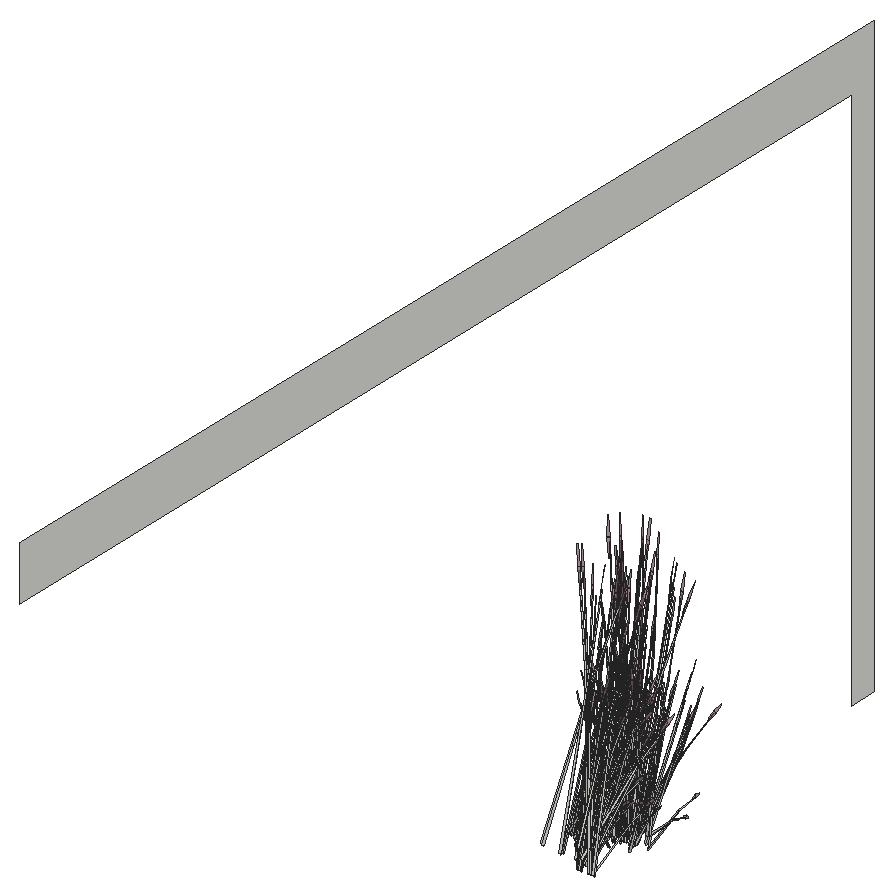
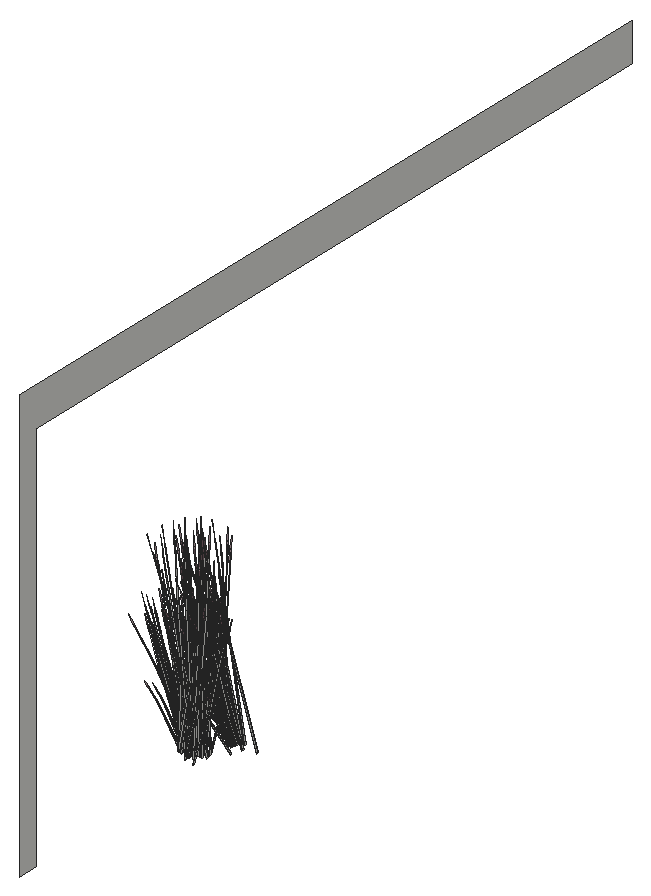
# SketchUp Ruby script. Lengths in inches.
U = 1.inch
M = Sketchup.active_model
def pt(a) = Geom::Point3d.new(a.map { |v| v * U })
def face(e, loops, mat)
  f = e.add_face(loops[0].map { |a| pt(a) })
  loops[1..].each { |l| e.add_face(l.map { |a| pt(a) }).erase! }
  f.material = f.back_material = mat if mat
  f
end
# faces: each face lists its corners as indices into pts; further lists are holes
def faces(e, pts, list, mat = nil) = list.each { |f| face(e, (f[0].is_a?(Array) ? f : [f]).map { |l| l.map { |i| pts[i] } }, mat) }
# xy, xz, yz: faces in a plane at the given z, y or x. An outline is a flat list of corners, or four numbers for a rectangle; further outlines are holes
def ring(l) = l.size == 4 ? [[l[0], l[1]], [l[2], l[1]], [l[2], l[3]], [l[0], l[3]]] : l.each_slice(2).to_a
def flat(e, list, mat, &to3) = list.each { |f| face(e, (f[0].is_a?(Array) ? f : [f]).map { |l| ring(l).map { |u, v| to3.(u, v) } }, mat) }
def xy(e, z, list, mat = nil) = flat(e, list, mat) { |x, y| [x, y, z] }
def xz(e, y, list, mat = nil) = flat(e, list, mat) { |x, z| [x, y, z] }
def yz(e, x, list, mat = nil) = flat(e, list, mat) { |y, z| [x, y, z] }
def lines(e, pts, list) = list.each { |a, b| e.add_line(pt(pts[a]), pt(pts[b])) }
# prism: a flat outline (further loops are holes) pulled along v
def prism(e, loops, v, mat = nil)
  f = face(e, loops, mat); d = Geom::Vector3d.new(v.map { |x| x * U })
  f.pushpull(f.normal.samedirection?(d) ? d.length : -d.length)
end
def box(e, o, s, mat = nil) = prism(e, [[o, [o[0] + s[0], o[1], o[2]], [o[0] + s[0], o[1] + s[1], o[2]], [o[0], o[1] + s[1], o[2]]]], [0, 0, s[2]], mat)
def at(x, y, z, deg = 0) = Geom::Transformation.translation(pt([x, y, z])) * Geom::Transformation.rotation(ORIGIN, Z_AXIS, deg.degrees)
def axes(o, x, y, z) = Geom::Transformation.new([*x, 0, *y, 0, *z, 0, *pt(o).to_a, 1])
def part(name) = M.definitions.add(name)
# library, detail: a bought-in or finely detailed component or shape, given as its bounding box
def library(name, o, s) = part(name).tap { |d| box(d.entities, o, s) }
def detail(e, o, s) = box(e.add_group.entities, o, s)
def put(e, d, t, mat = nil) = e.add_instance(d, t).tap { |i| i.material = mat if mat }
def group(e, t, mat = nil) = e.add_group.tap { |g| g.transformation = t; g.material = mat if mat }.entities
root = M.entities
M.materials.add("LightPink_Translucent").color = [144, 107, 117]
M.materials["LightPink_Translucent"].alpha = 0.75
c1 = part("blade")
p = [[2.15,0.21,22],[0,0.17,0],[0.09,0.45,0],[2.18,0.31,22],[2.29,0.31,22],[0.38,0.45,0],
  [2.48,0.24,33],[2.49,0.24,33],[2.48,0.22,33]]
faces(c1.entities,p,[[0,1,2,3],[4,5,2,3],[6,3,4,7],[8,0,3,6]])
c2 = part("seeds")
p = [[0.3,-0.1,1.38],[-0.01,-0.03,1.59],[-0.01,-0.03,0.03],[0.14,-0.07,-0.07],[0.29,-0.03,3],[0.15,0.01,3.11]]
faces(c2.entities,p,[[0,1,2,3],[1,0,4,5]],"LightPink_Translucent")
c3 = part("blade with seeds")
put(c3.entities,c1,at(0,0,0))
put(c3.entities,c2,axes([2.4,0.25,30.99],[1.5799,-0.05474,1.17369],[-0.12525,1.92788,0.29478],[-0.07173,-0.02425,1.56792]))
yz(root,294,[[525,0,531,0,531,132,297,132,297,120,525,120]])
put(root,c3,axes([298.87,447.625,2.375],[1.11865,0,0],[0,0.72922,-0.51607],[0,0.16609,1.63711]))
put(root,c3,axes([298.43,448,2.2],[-1.1181,-0.00522,-0.04976],[0,-0.72922,0.49943],[-0.03514,0.166,1.58352]))
put(root,c3,axes([296.01,447.37,2.67],[1.00749,0.31132,-0.29095],[-0.48511,0.65709,-0.50002],[0.03166,0.16133,1.59708]))
put(root,c3,axes([290.6875,453.29,5.03],[-0.45012,-0.59081,-0.1216],[0.79888,-0.29033,-0.67495],[0.33665,-0.07795,1.02557]))
put(root,c3,axes([297.95,449.24,4.53],[0.50902,0.40851,-0.35414],[-0.58122,0.38671,0.4572],[0.29531,0.05884,0.87481]))
put(root,c3,axes([298.19,448.11,2.03],[-0.62448,0.40708,-0.30978],[-0.62448,-0.40708,0.30978],[0,0.13112,1.38974]))
put(root,c3,axes([290.65,452.79,4.68],[0.24236,-0.59349,-0.51099],[0.83094,0.20343,-0.3958],[0.33455,-0.05442,0.97773]))
put(root,c3,axes([289.33,450.37,2.375],[0.55932,-0.6538,0],[0.93577,0.36461,-0.51607],[0.21313,0.08304,1.63711]))
put(root,c3,axes([297.6875,449.4,4.73],[-0.04505,0.49615,0.0643],[-0.68022,-0.0136,0.50621],[0.26056,0.05192,0.77189]))
put(root,c3,axes([295.9,447.85,2.21],[-0.43405,0.58792,-0.44739],[-0.90188,-0.28295,0.21531],[0,0.13553,1.43643]))
put(root,c3,axes([297.75,449.24,4.73],[-0.65964,0.42992,0.48003],[-0.5689,-0.45657,0.3958],[0.30948,0.0793,0.9933]))
put(root,c3,axes([291.54,452.95,1.98],[-0.57619,0.0783,1.41583],[-0.09171,-0.62326,0.08104],[0.40356,-0.09434,0.80566]))
put(root,c3,axes([292.58,452.4,2.26],[-0.55463,-0.41721,-0.06488],[0.60744,-0.38228,-0.29416],[0.17212,-0.02691,0.97024]))
put(root,c3,axes([290.49,453,4.98],[0.78611,-0.28816,-0.71045],[0.4381,0.59317,0.08574],[0.37982,-0.06738,1.00501]))
put(root,c3,axes([295.65,449.74,5.05],[-0.13817,-0.52554,0.35414],[0.78985,-0.13877,-0.4572],[0.21215,0.1506,0.87481]))
put(root,c3,axes([295.92,449.54,2.33],[1.11998,0.21207,0.30756],[-0.2802,0.75803,-0.36492],[-0.18537,0.09487,1.64885]))
put(root,c3,axes([298.62,448.12,2.02],[0,0.65246,-0.49651],[-1.00089,0,0],[0,0.1486,1.57504]))
put(root,c3,axes([296.12,448.19,3.875],[-0.3323,-0.11241,1.71376],[0.68769,-0.4716,0.13857],[0.42861,0.21275,0.73262]))
put(root,c3,axes([290.375,453.12,5.05],[-0.74348,-0.18202,0.35414],[0.21685,-0.53102,-0.4572],[0.29933,-0.04869,0.87481]))
put(root,c3,axes([296.18,446.71,4.47],[-0.77304,-0.33901,1.38283],[0.81626,-0.52782,0.59665],[0.24941,0.31809,1.33663]))
put(root,c3,axes([285.29,451.53,1.59],[-0.88056,0.26122,1.28929],[-0.28027,-0.74951,0.50096],[0.54072,0.01247,1.46642]))
put(root,c3,axes([297.35,449.47,2.77],[-0.5037,-0.18761,1.1486],[0.6504,-0.19062,0.84392],[0.17543,0.16147,0.25299]))
put(root,c3,axes([295.58,450.01,5.03],[0.53309,-0.55848,-0.1216],[0.77201,0.32175,-0.67495],[0.26836,0.15779,1.02557]))
put(root,c3,axes([292.16,452.55,1.49],[-0.04675,-0.09906,1.76342],[0.32428,-0.57943,-0.26939],[0.32711,-0.00833,0.30037]))
put(root,c3,axes([296.6,449.95,2.375],[0.55932,0.6538,0],[-0.93577,0.36461,-0.51607],[-0.21313,0.08304,1.63711]))
put(root,c3,axes([294.88,450.47,4.71],[0.00265,-0.07899,1.77383],[0.76665,-0.34851,-0.16761],[0.2663,0.12439,0.31391]))
put(root,c3,axes([291.16,453.06,4.53],[0.74348,0.18202,-0.35414],[-0.21685,0.53102,0.4572],[0.29933,-0.04869,0.87481]))
put(root,c3,axes([297.49,450.17,1.49],[0.06518,-0.0942,1.76342],[0.82057,-0.27742,-0.26939],[0.24877,0.14358,0.30037]))
put(root,c3,axes([296.41,448.03,2.09],[0.32803,0.59738,-0.69212],[-0.94492,0.21515,-0.18165],[0.03626,0.20229,1.52773]))
put(root,c3,axes([296.21,449.73,4.68],[0.88277,-0.1551,-0.51099],[0.15442,0.58737,-0.3958],[0.23711,0.16832,0.97773]))
put(root,c3,axes([289.84,450.76,2.02],[0.83726,0.32623,-0.49651],[-0.50045,0.58498,0],[0.19069,0.0743,1.57504]))
put(root,c3,axes([293.76,449.82,5.05],[0.2697,-0.50175,0.35414],[0.78684,0.14635,-0.4572],[0.07215,0.20201,0.87481]))
put(root,c3,axes([297.43,450.33,2.67],[-0.57368,-0.02046,1.0506],[0.37886,-0.43461,0.58006],[0.22663,0.15441,0.8241]))
put(root,c3,axes([289.13,452.4,3.875],[-0.37107,0.01478,1.71376],[0.24616,-0.64047,0.13857],[0.5288,0.03961,0.73262]))
put(root,c3,axes([295.78,450.21,4.73],[-0.4066,0.41448,0.0643],[-0.57901,-0.24131,0.50621],[0.18719,0.13288,0.77189]))
put(root,c3,axes([291.05,453.28,4.73],[0.32857,0.44488,0.0643],[-0.59916,0.21775,0.50621],[0.26412,-0.04296,0.77189]))
put(root,c3,axes([294.82,451.61,5.65],[0.61821,-0.37431,-0.06488],[0.56645,0.40995,-0.29416],[0.03988,0.11616,0.97024]))
put(root,c3,axes([290.98,453.125,4.73],[-0.25275,0.59491,0.48003],[-0.83094,-0.20343,0.3958],[0.32677,-0.03575,0.9933]))
put(root,c3,axes([295.95,450.1,4.73],[-0.88979,0.14973,0.48003],[-0.15442,-0.58737,0.3958],[0.20926,0.17311,0.9933]))
put(root,c3,axes([295.56,449.27,2.59],[0.01579,-0.21629,1.43002],[0.75442,-0.24159,-0.30754],[0.23289,0.25887,0.61141]))
put(root,c3,axes([293.52,450.28,4.73],[-0.6592,0.22175,0.0643],[-0.32265,-0.40436,0.50621],[0.06366,0.17825,0.77189]))
put(root,c3,axes([288.62,452.01,2.06],[0.9306,0.10697,-0.62353],[-0.19638,0.65984,-0.16365],[0.27771,0.07995,1.37633]))
put(root,c3,axes([292.73,453.17,2.77],[-0.55274,0.10771,1.1486],[0.26018,-0.44517,0.84392],[0.29323,0.03046,0.25299]))
put(root,c3,axes([293.5,450.03,5.03],[0.87543,-0.30377,-0.1216],[0.4302,0.53915,-0.67495],[0.1155,0.2272,1.02557]))
put(root,c3,axes([293.75,450.23,5.0625],[-0.88151,-0.17057,0.53283],[0.30143,-0.56078,0.43934],[0.05297,0.22053,1.10256]))
put(root,c3,axes([296.2,459.12,2.59],[-0.25429,0.13207,1.43002],[-0.76157,-0.23115,-0.30754],[0.14117,-0.28747,0.61141]))
put(root,c3,axes([293.66,450.15,1.49],[0.14478,-0.0355,1.76342],[0.8709,0.19542,-0.26939],[0.02547,0.22025,0.30037]))
put(root,c3,axes([292.48,455.05,4.71],[-0.08089,-0.05712,1.77383],[0.17695,-0.61228,-0.16761],[0.31864,-0.03912,0.31391]))
put(root,c3,axes([291.77,454.54,3.93],[-0.17122,-0.54847,-0.03492],[0.80929,-0.12609,-0.15832],[0.169,0.03477,0.52218]))
put(root,c3,axes([294.31,458.4,1.49],[-0.15005,0.02351,1.76342],[-0.82981,-0.26461,-0.26939],[0.01392,-0.22072,0.30037]))
put(root,c3,axes([289.68,454.52,5.03],[0.0479,-0.66354,-0.1216],[0.90696,0.01814,-0.67495],[0.3493,0.04609,1.02557]))
put(root,c3,axes([294.25,450.01,4.68],[0.87941,0.16356,-0.51099],[-0.30143,0.56078,-0.3958],[0.08064,0.22578,0.97773]))
put(root,c3,axes([294.75,448.85,3.875],[-0.2045,-0.20949,1.71376],[0.94495,-0.17636,0.13857],[0.21357,0.32887,0.73262]))
put(root,c3,axes([296.82,460.1,4.98],[0.02328,-0.60353,-0.71045],[0.98022,0.04053,0.08574],[0.10344,-0.25568,1.00501]))
put(root,c3,axes([289.54,454.26,5.05],[-0.50902,-0.40851,0.35414],[0.58122,-0.38671,-0.4572],[0.29531,0.05884,0.87481]))
put(root,c3,axes([293.85,450.35,4.53],[-0.2697,0.50175,-0.35414],[-0.78684,-0.14635,0.4572],[0.07215,0.20201,0.87481]))
put(root,c3,axes([298.1875,459.15,4.72],[-0.00864,-0.12985,1.74944],[-0.72937,-0.3753,-0.27667],[0.11277,-0.2275,0.14031]))
put(root,c3,axes([295.125,459.125,4.53],[0.2697,-0.50175,-0.35414],[0.78684,0.14635,0.4572],[-0.07215,-0.20201,0.87481]))
put(root,c3,axes([295.72,459.79,3.875],[-0.16657,0.22426,1.71376],[-0.69879,-0.4641,0.13857],[0.31524,-0.28926,0.73262]))
put(root,c3,axes([297.99,458.6875,4.71],[-0.09085,0.04984,1.77383],[-0.89014,-0.16814,-0.16761],[-0.03222,-0.21748,0.31391]))
put(root,c3,axes([291.7,453.88,2.59],[-0.21545,-0.16047,1.43002],[0.28033,-0.53085,-0.30754],[0.43591,0.07191,0.61141]))
put(root,c3,axes([295.27,458.07,2.77],[0.11476,0.38047,1.1486],[-0.63664,-0.21072,0.84392],[0.06851,-0.19481,0.25299]))
put(root,c3,axes([296.62,459.89,4.68],[-0.64041,-0.4384,-0.51099],[0.67652,-0.38394,-0.3958],[0.09744,-0.22274,0.97773]))
put(root,c3,axes([290.46,454.125,4.72],[0.19191,-0.01103,1.74944],[0.52639,-0.5069,-0.27667],[0.34136,0.06691,0.14031]))
put(root,c3,axes([293.93,449.9,4.98],[0.42698,0.53052,-0.71045],[-0.87893,0.29566,0.08574],[0.09984,0.25633,1.00501]))
put(root,c3,axes([293.29,451.24,4.72],[0.1134,0.10507,1.74944],[0.91515,0.04128,-0.27667],[0.09203,0.23172,0.14031]))
put(root,c3,axes([295.22,459.24,4.73],[0.88151,0.17057,0.48003],[-0.30143,0.56078,0.3958],[-0.05297,-0.22053,0.9933]))
put(root,c3,axes([289.72,454.2,4.98],[0.89428,0.01571,-0.71045],[-0.06006,0.66153,0.08574],[0.37886,0.06981,1.00501]))
put(root,c3,axes([297.29,460.125,5.03],[-0.98321,-0.03233,-0.1216],[0.02687,-0.61208,-0.67495],[0.0683,-0.23574,1.02557]))
put(root,c3,axes([297.22,459.73,4.53],[0.60531,-0.34352,-0.35414],[0.573,0.39225,0.4572],[0.08718,-0.19929,0.87481]))
put(root,c3,axes([295.45,459.2,4.73],[0.6592,-0.22175,0.0643],[0.32265,0.40436,0.50621],[-0.06366,-0.17825,0.77189]))
put(root,c3,axes([290.26,454.48,4.53],[0.50902,0.40851,-0.35414],[-0.58122,0.38671,0.4572],[0.29531,0.05884,0.87481]))
put(root,c3,axes([290,454.63,4.73],[-0.04505,0.49615,0.0643],[-0.68022,-0.0136,0.50621],[0.26056,0.05192,0.77189]))
put(root,c3,axes([290.06,454.47,4.73],[-0.65964,0.42992,0.48003],[-0.5689,-0.45657,0.3958],[0.30948,0.0793,0.9933]))
put(root,c3,axes([297.98,459.52,1.49],[-0.1339,-0.0514,1.76342],[-0.34394,-0.57425,-0.26939],[0.23202,-0.15583,0.30037]))
put(root,c3,axes([295.21,459.65,5.05],[-0.2697,0.50175,0.35414],[-0.78684,-0.14635,-0.4572],[-0.07215,-0.20201,0.87481]))
put(root,c3,axes([297.22,459.87,4.73],[0.63704,0.44518,0.48003],[-0.67652,0.38394,0.3958],[0.11751,-0.20886,0.9933]))
put(root,c3,axes([297.46,459.91,4.73],[0.73517,0.0304,0.0643],[-0.02016,0.45906,0.50621],[0.07693,-0.17585,0.77189]))
put(root,c3,axes([288.43,453.43,3.875],[-0.3323,-0.11241,1.71376],[0.68769,-0.4716,0.13857],[0.42861,0.21275,0.73262]))
put(root,c3,axes([296.91,460.22,5.05],[-0.60531,0.34352,0.35414],[-0.573,-0.39225,-0.4572],[0.08718,-0.19929,0.87481]))
put(root,c3,axes([297.98,461.14,4.98],[0.4673,-0.51481,-0.71045],[0.81887,0.36587,0.08574],[0.27902,-0.18652,1.00501]))
put(root,c3,axes([292.92,459.65,2.375],[-0.55932,-0.6538,0],[0.93577,-0.36461,-0.51607],[0.21313,-0.08304,1.63711]))
put(root,c3,axes([297.95,460.9,4.68],[-0.22982,-0.59576,-0.51099],[0.87033,-0.10422,-0.3958],[0.24941,-0.16002,0.97773]))
put(root,c3,axes([287.89,455.24,5.03],[0.53309,-0.55848,-0.1216],[0.77201,0.32175,-0.67495],[0.26836,0.15779,1.02557]))
put(root,c3,axes([298.36,461.33,5.03],[-0.82753,-0.35977,-0.1216],[0.47675,-0.52101,-0.67495],[0.2338,-0.18111,1.02557]))
put(root,c3,axes([289.8,455.41,1.49],[0.06518,-0.0942,1.76342],[0.82057,-0.27742,-0.26939],[0.24877,0.14358,0.30037]))
put(root,c3,axes([293.68,459.54,2.02],[0.83726,-0.32623,-0.49651],[0.50045,0.58498,0],[0.19069,-0.0743,1.57504]))
put(root,c3,axes([298.65,460.67,2.59],[-0.31959,-0.01933,1.43002],[-0.32741,-0.51843,-0.30754],[0.39262,-0.14666,0.61141]))
put(root,c3,axes([300.4,461.17,4.71],[-0.11685,-0.00496,1.77383],[-0.48522,-0.53096,-0.16761],[0.19486,-0.17458,0.31391]))
put(root,c3,axes([288.52,454.97,4.68],[0.88277,-0.1551,-0.51099],[0.15442,0.58737,-0.3958],[0.23711,0.16832,0.97773]))
put(root,c3,axes([294.68,460.88,2.06],[0.60257,-0.49041,-0.62353],[0.74854,0.44469,-0.16365],[0.24146,-0.12234,1.37633]))
put(root,c3,axes([299.02,459.72,2.77],[-0.29798,0.33213,1.1486],[-0.25612,-0.44624,0.84392],[0.24611,-0.11182,0.25299]))
put(root,c3,axes([298.59,460.97,4.53],[0.77872,-0.09325,-0.35414],[0.20563,0.53305,0.4572],[0.22316,-0.14318,0.87481]))
put(root,c3,axes([293.625,461.74,2.21],[0.43405,-0.58792,-0.44739],[0.90188,0.28295,0.21531],[0,-0.13553,1.43643]))
put(root,c3,axes([294.02,461.45,2.67],[-0.10425,-0.7445,-0.29095],[1.08575,-0.04502,-0.50002],[0.19119,-0.09917,1.59708]))
put(root,c3,axes([297.96,461.28,5.05],[-0.77872,0.09325,0.35414],[-0.20563,-0.53305,-0.4572],[0.22316,-0.14318,0.87481]))
put(root,c3,axes([293.88,459.8,2.03],[0.83462,0.16144,-0.30978],[-0.21015,0.56852,0.30978],[0.16826,-0.06556,1.38974]))
put(root,c3,axes([298.66,461.2,4.73],[0.61415,0.2744,0.0643],[-0.35756,0.39076,0.50621],[0.1969,-0.12633,0.77189]))
put(root,c3,axes([298.49,461.08,4.73],[0.22187,0.60049,0.48003],[-0.87033,0.10422,0.3958],[0.25651,-0.14123,0.9933]))
put(root,c3,axes([300.84,461.81,4.72],[0.12414,-0.09938,1.74944],[-0.15889,-0.60963,-0.27667],[0.31148,-0.11559,0.14031]))
put(root,c3,axes([294.16,462.03,2.43],[1.00799,0.31623,0.24065],[-0.48511,0.65709,0.50002],[0,-0.15147,1.60543]))
put(root,c3,axes([293.84,461.59,2.72],[-0.97146,0.04028,0.44739],[-0.08785,-0.66859,-0.21531],[0.17391,-0.06776,1.43643]))
put(root,c3,axes([298.4,462.73,5.03],[-0.45012,-0.59081,-0.1216],[0.79888,-0.29033,-0.67495],[0.33665,-0.07795,1.02557]))
put(root,c3,axes([298.36,462.23,4.68],[0.24236,-0.59349,-0.51099],[0.83094,0.20343,-0.3958],[0.33455,-0.05442,0.97773]))
put(root,c3,axes([297.04,459.81,2.375],[0.55932,-0.6538,0],[0.93577,0.36461,-0.51607],[0.21313,0.08304,1.63711]))
put(root,c3,axes([293.81,461.83,2.36],[0.38895,0.72959,0.45755],[-1.11135,0.2537,0.17955],[0.01358,-0.13406,1.58856]))
put(root,c3,axes([296.1,465.625,2.59],[-0.25429,0.13207,1.43002],[-0.76157,-0.23115,-0.30754],[0.14117,-0.28747,0.61141]))
put(root,c3,axes([299.24,462.39,1.98],[-0.57619,0.0783,1.41583],[-0.09171,-0.62326,0.08104],[0.40356,-0.09434,0.80566]))
put(root,c3,axes([300.29,461.84,2.26],[-0.55463,-0.41721,-0.06488],[0.60744,-0.38228,-0.29416],[0.17212,-0.02691,0.97024]))
put(root,c3,axes([295.2,461.9,2.21],[0,-0.75495,0],[1.11865,0,0],[0,0,1.79456]))
put(root,c3,axes([294.21,464.91,1.49],[-0.15005,0.02351,1.76342],[-0.82981,-0.26461,-0.26939],[0.01392,-0.22072,0.30037]))
put(root,c3,axes([296.56,460.15,2.48],[-0.83726,-0.32623,0.49651],[0.50045,-0.58498,0],[0.19069,0.0743,1.57504]))
put(root,c3,axes([298.2,462.44,4.98],[0.78611,-0.28816,-0.71045],[0.4381,0.59317,0.08574],[0.37982,-0.06738,1.00501]))
put(root,c3,axes([294.67,461.42,2.36],[-0.74176,0.59212,0.45755],[-0.88124,-0.52269,0.17955],[0.17882,-0.05909,1.58856]))
put(root,c3,axes([296.72,466.6,4.98],[0.02328,-0.60353,-0.71045],[0.98022,0.04053,0.08574],[0.10344,-0.25568,1.00501]))
put(root,c3,axes([295.48,462.48,2.3],[-0.83213,-0.56158,-0.06131],[0.83263,-0.56193,0],[-0.02906,-0.01961,1.75571]))
put(root,c3,axes([298.09,465.66,4.72],[-0.00864,-0.12985,1.74944],[-0.72937,-0.3753,-0.27667],[0.11277,-0.2275,0.14031]))
put(root,c3,axes([295.02,465.63,4.53],[0.2697,-0.50175,-0.35414],[0.78684,0.14635,0.4572],[-0.07215,-0.20201,0.87481]))
put(root,c3,axes([293.39,460.45,2.47],[-0.25843,0.64844,0.17642],[-0.9457,-0.1835,0.35086],[0.16336,-0.00316,1.60407]))
put(root,c3,axes([295.62,466.3,3.875],[-0.16657,0.22426,1.71376],[-0.69879,-0.4641,0.13857],[0.31524,-0.28926,0.73262]))
put(root,c3,axes([297.89,465.19,4.71],[-0.09085,0.04984,1.77383],[-0.89014,-0.16814,-0.16761],[-0.03222,-0.21748,0.31391]))
put(root,c3,axes([298.08,462.56,5.05],[-0.74348,-0.18202,0.35414],[0.21685,-0.53102,-0.4572],[0.29933,-0.04869,0.87481]))
put(root,c3,axes([293,460.97,1.59],[-0.88056,0.26122,1.28929],[-0.28027,-0.74951,0.50096],[0.54072,0.01247,1.46642]))
put(root,c3,axes([295.36,461.17,2.62],[0.17258,-0.58229,0.1448],[0.84319,0.10108,-0.41347],[0.15345,0.05979,1.26744]))
put(root,c3,axes([295.17,464.57,2.77],[0.11476,0.38047,1.1486],[-0.63664,-0.21072,0.84392],[0.06851,-0.19481,0.25299]))
put(root,c3,axes([299.87,461.99,1.49],[-0.04675,-0.09906,1.76342],[0.32428,-0.57943,-0.26939],[0.32711,-0.00833,0.30037]))
put(root,c3,axes([296.52,466.4,4.68],[-0.64041,-0.4384,-0.51099],[0.67652,-0.38394,-0.3958],[0.09744,-0.22274,0.97773]))
put(root,c3,axes([295,461.32,2.72],[-0.53742,-0.54764,0.44739],[0.81403,-0.38564,-0.21531],[0.17391,0.06776,1.43643]))
put(root,c3,axes([295.28,461.36,2.67],[0.90324,-0.43318,-0.29095],[0.60064,0.61207,-0.50002],[0.22285,0.06216,1.59708]))
put(root,c3,axes([298.87,462.5,4.53],[0.74348,0.18202,-0.35414],[-0.21685,0.53102,0.4572],[0.29933,-0.04869,0.87481]))
put(root,c3,axes([295.12,465.75,4.73],[0.88151,0.17057,0.48003],[-0.30143,0.56078,0.3958],[-0.05297,-0.22053,0.9933]))
put(root,c3,axes([297.55,460.2,2.02],[0.83726,0.32623,-0.49651],[-0.50045,0.58498,0],[0.19069,0.0743,1.57504]))
put(root,c3,axes([297.19,466.63,5.03],[-0.98321,-0.03233,-0.1216],[0.02687,-0.61208,-0.67495],[0.0683,-0.23574,1.02557]))
put(root,c3,axes([295.96,462.06,2.21],[1.00089,0,0],[0,0.67548,0],[0,0,1.78407]))
put(root,c3,axes([297.125,466.24,4.53],[0.60531,-0.34352,-0.35414],[0.573,0.39225,0.4572],[0.08718,-0.19929,0.87481]))
put(root,c3,axes([295.36,465.71,4.73],[0.6592,-0.22175,0.0643],[0.32265,0.40436,0.50621],[-0.06366,-0.17825,0.77189]))
put(root,c3,axes([296.25,460.48,2.47],[-0.96132,0.17317,0.17642],[-0.23737,-0.64447,0.35086],[0.08574,0.0939,1.60407]))
put(root,c3,axes([296.84,461.84,3.875],[-0.37107,0.01478,1.71376],[0.24616,-0.64047,0.13857],[0.5288,0.03961,0.73262]))
put(root,c3,axes([297.32,460.45,2.03],[0.21015,0.56852,-0.30978],[-0.83462,0.16144,0.30978],[0.16826,0.06556,1.38974]))
put(root,c3,axes([298.76,462.72,4.73],[0.32857,0.44488,0.0643],[-0.59916,0.21775,0.50621],[0.26412,-0.04296,0.77189]))
put(root,c3,axes([295.64,461.72,2.38],[-1.13071,-0.13747,0.49198],[0.23011,-0.77639,0.19306],[0.16524,0.07497,1.70813]))
put(root,c3,axes([298.69,462.5625,4.73],[-0.25275,0.59491,0.48003],[-0.83094,-0.20343,0.3958],[0.32677,-0.03575,0.9933]))
put(root,c3,axes([294.74,463.64,2.2],[-0.29189,-0.56252,0],[0.83351,-0.19699,0],[0,0,1.54371]))
put(root,c3,axes([295.83,463.56,2.18],[0.93921,-0.22138,-0.19198],[0.33003,0.6377,0.00008],[0.10367,-0.02447,1.73897]))
